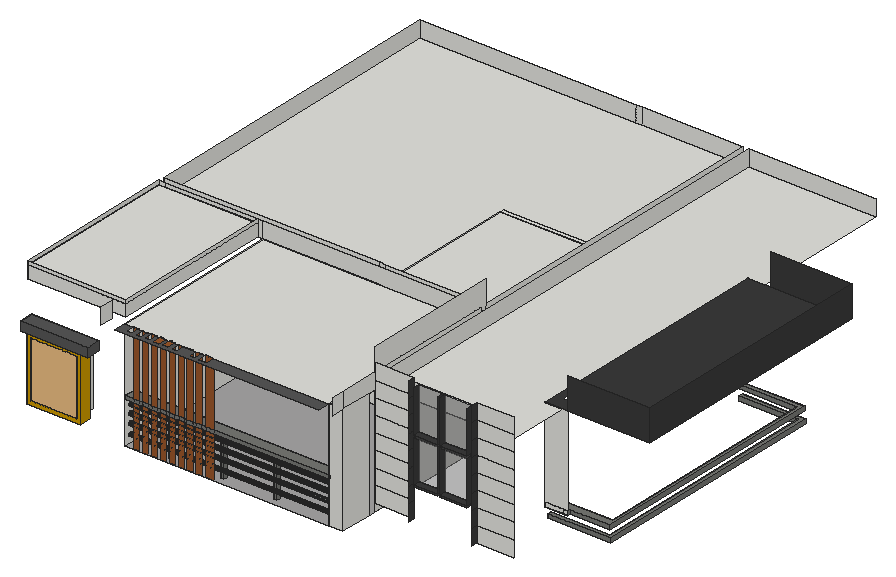
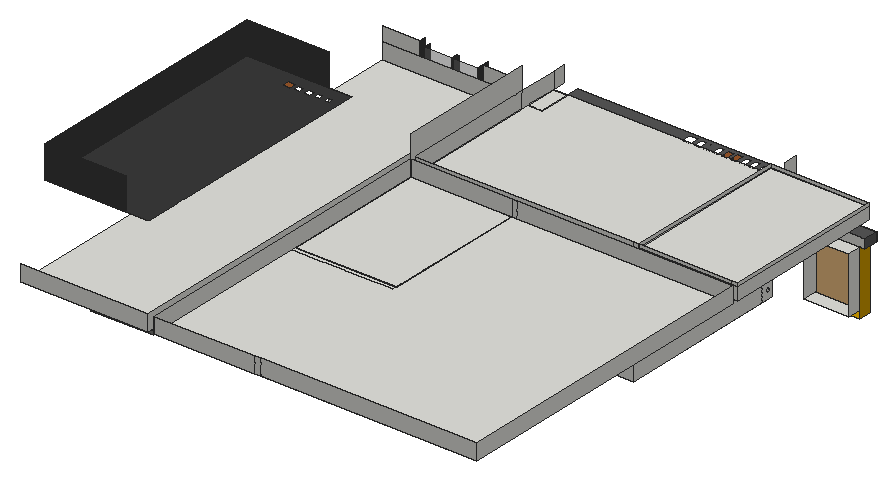
# SketchUp Ruby script. Lengths in inches.
U = 1.inch
M = Sketchup.active_model
def pt(a) = Geom::Point3d.new(a.map { |v| v * U })
def face(e, loops, mat)
  f = e.add_face(loops[0].map { |a| pt(a) })
  loops[1..].each { |l| e.add_face(l.map { |a| pt(a) }).erase! }
  f.material = f.back_material = mat if mat
  f
end
# faces: each face lists its corners as indices into pts; further lists are holes
def faces(e, pts, list, mat = nil) = list.each { |f| face(e, (f[0].is_a?(Array) ? f : [f]).map { |l| l.map { |i| pts[i] } }, mat) }
# xy, xz, yz: faces in a plane at the given z, y or x. An outline is a flat list of corners, or four numbers for a rectangle; further outlines are holes
def ring(l) = l.size == 4 ? [[l[0], l[1]], [l[2], l[1]], [l[2], l[3]], [l[0], l[3]]] : l.each_slice(2).to_a
def flat(e, list, mat, &to3) = list.each { |f| face(e, (f[0].is_a?(Array) ? f : [f]).map { |l| ring(l).map { |u, v| to3.(u, v) } }, mat) }
def xy(e, z, list, mat = nil) = flat(e, list, mat) { |x, y| [x, y, z] }
def xz(e, y, list, mat = nil) = flat(e, list, mat) { |x, z| [x, y, z] }
def yz(e, x, list, mat = nil) = flat(e, list, mat) { |y, z| [x, y, z] }
def lines(e, pts, list) = list.each { |a, b| e.add_line(pt(pts[a]), pt(pts[b])) }
# prism: a flat outline (further loops are holes) pulled along v
def prism(e, loops, v, mat = nil)
  f = face(e, loops, mat); d = Geom::Vector3d.new(v.map { |x| x * U })
  f.pushpull(f.normal.samedirection?(d) ? d.length : -d.length)
end
def box(e, o, s, mat = nil) = prism(e, [[o, [o[0] + s[0], o[1], o[2]], [o[0] + s[0], o[1] + s[1], o[2]], [o[0], o[1] + s[1], o[2]]]], [0, 0, s[2]], mat)
def at(x, y, z, deg = 0) = Geom::Transformation.translation(pt([x, y, z])) * Geom::Transformation.rotation(ORIGIN, Z_AXIS, deg.degrees)
def axes(o, x, y, z) = Geom::Transformation.new([*x, 0, *y, 0, *z, 0, *pt(o).to_a, 1])
def part(name) = M.definitions.add(name)
# library, detail: a bought-in or finely detailed component or shape, given as its bounding box
def library(name, o, s) = part(name).tap { |d| box(d.entities, o, s) }
def detail(e, o, s) = box(e.add_group.entities, o, s)
def put(e, d, t, mat = nil) = e.add_instance(d, t).tap { |i| i.material = mat if mat }
def group(e, t, mat = nil) = e.add_group.tap { |g| g.transformation = t; g.material = mat if mat }.entities
root = M.entities
M.materials.add("[Color C05]").color = [255, 93, 0]
M.materials.add("[Color C08]").color = [74, 47, 0]
M.materials.add("[Color D06]").color = [204, 153, 0]
M.materials.add("[Color M06]").color = [86, 86, 86]
M.materials.add("[Color M07]").color = [58, 58, 58]
M.materials.add("[Metal Seamed]").color = [118, 119, 115]
M.materials.add("[Stone Vein Gray]").color = [166, 165, 165]
M.materials.add("[Translucent Glass Gray]").color = [128, 128, 128]
M.materials["[Translucent Glass Gray]"].alpha = 0.5
M.materials.add("[Wood Cherry Original]").color = [152, 86, 42]
c1 = part("Group\#3")
xy(c1.entities,0,[[0,0,48,8.5625]],"[Color C08]")
xy(c1.entities,4.98,[[4.98,0,43.02,2.5625],[4.98,2.5625,43.02,8.5625]],"[Color C08]")
xy(c1.entities,79.02,[[4.98,0,43.02,2.5625],[4.98,2.5625,43.02,8.5625]],"[Color C08]")
xy(c1.entities,84,[[0,0,48,8.5625]],"[Color C08]")
xz(c1.entities,0,[[[0,0,48,84],[4.98,4.98,43.02,79.02]]],"[Color C08]")
xz(c1.entities,2.5625,[[4.98,4.98,43.02,79.02]],"[Color C05]")
xz(c1.entities,8.5625,[[[0,0,48,84],[4.98,4.98,43.02,79.02]]],"[Color C08]")
yz(c1.entities,0,[[0,0,8.5625,84]],"[Color C08]")
yz(c1.entities,4.98,[[0,4.98,2.5625,79.02],[2.5625,4.98,8.5625,79.02]],"[Color C08]")
yz(c1.entities,43.02,[[0,4.98,2.5625,79.02],[2.5625,4.98,8.5625,79.02]],"[Color C08]")
yz(c1.entities,48,[[0,0,8.5625,84]],"[Color C08]")
c2 = library("Group\#4",[0,0,0],[48,6,60])
xy(root,164.875,[[336.97,106.4375,352,140.0625]])
xy(root,164.875,[[273.15,113.09,276.47,116.4]],"[Metal Seamed]")
xy(root,164.875,[[[120,106.4375,336.97,106.4375,336.97,140.0625,352,140.0625,352,449.1875,322.29,449.1875,322.29,453.4375,274.29,453.4375,274.29,449.1875,244.75,449.1875,244.75,290.0625,120,290.0625],[161.28,113.09,164.59,116.4],[216.4,113.09,219.72,116.4],[273.15,113.09,276.47,116.4]]],"[Stone Vein Gray]")
xy(root,169.04,[[475.4375,224.05,475.4375,228.48,537.83,228.48,537.83,478.41,475.4375,478.41,475.4375,483.17,542.5625,483.17,542.5625,224.05]],"[Metal Seamed]")
xy(root,173.48,[[475.4375,224.05,542.5625,224.05,542.5625,483.17,475.4375,483.17,475.4375,478.41,537.83,478.41,537.83,228.48,475.4375,228.48]],"[Metal Seamed]")
xy(root,176.87,[[25.93,93.75,82.74,106.4375]],"[Color D06]")
xy(root,179.95,[[180.25,290.0625,233.4375,296.0625]])
xy(root,181.27,[[30.34,93.75,78.34,115.4375]])
xy(root,181.87,[[475.4375,220.28,475.4375,231.31,538.41,231.31,538.41,476.42,541.89,476.42,541.89,481.18,542.5625,481.18,542.5625,222.97,500,222.97,500,220.28],[475.4375,476.33,475.4375,481.18,534.52,481.18,534.52,480.67,536.58,480.67,536.58,476.33],[536.58,476.33,538.41,476.42],[536.58,476.42,541.89,480.67],[534.52,480.67,541.89,481.18]],"[Metal Seamed]")
xy(root,182.4375,[[536.02,226.32,541.65,232.26]],"[Metal Seamed]")
xy(root,186.3125,[[475.4375,220.28,500,220.28,500,222.97,542.5625,222.97,542.5625,481.18,475.4375,481.18,475.4375,476.33,538.41,476.33,538.41,231.31,475.4375,231.31]],"[Metal Seamed]")
xy(root,208.4375,[[216.4,113.09,219.72,116.4]],"[Metal Seamed]")
xy(root,208.53,[[399.25,141.23,424.3125,147.79],[427.08,141.23,456,147.79]],"[Color M07]")
xy(root,209.16,[[336.97,106.4375,337.375,118.875],[336.97,118.875,337.375,140.0625]])
xy(root,209.16,[[[120,106.4375,336.97,118.875],[161.28,113.09,164.59,116.4],[273.15,113.09,276.47,116.4]]],"[Metal Seamed]")
xy(root,210.6,[[399.25,141.23,424.3125,147.79],[427.08,141.23,456,147.79]],"[Color M07]")
xy(root,212.875,[[336.97,106.4375,337.375,118.875],[336.97,118.875,337.375,140.0625]])
xy(root,212.875,[[120,106.4375,336.97,118.875]],"[Metal Seamed]")
xy(root,241.27,[[30.34,93.75,78.34,115.4375]])
xy(root,245.68,[[25.93,93.75,82.74,106.4375]])
xy(root,245.68,[[20.68,91.3125,20.68,106.4375,25.93,106.4375,25.93,93.75,82.74,93.75,82.74,106.4375,92.11,106.4375,92.11,91.3125]],"[Color M06]")
xy(root,248.875,[[274.29,449.1875,322.29,453.4375]])
xy(root,251.14,[[180.25,290.0625,233.4375,296.0625]])
xy(root,255.3,[[20.68,91.3125,92.11,106.4375]],"[Color M06]")
xy(root,255.4,[[399.25,141.23,424.3125,147.79],[427.08,141.23,456,147.79]],"[Color M07]")
xy(root,257.48,[[399.25,141.23,424.3125,147.79],[427.08,141.23,456,147.79]],"[Color M07]")
xy(root,280.8125,[[186.11,97.4375,191.67,106.4375]],"[Wood Cherry Original]")
xy(root,281,[[120,106.4375,120,290.0625,352,290.0625,352,140.0625,336.97,140.0625,336.97,106.4375],[336.97,106.4375,352,140.0625],[358,155.92,494,155.92,494,220.28,475.4375,220.28,475.4375,489.49,494,489.49,494,637.4375,358,637.4375],[244.75,290.0625,352,296.0625],[9,296.0625,244.75,296.0625,244.75,453.4375,352,453.4375,352,637.4375,9,637.4375],
  [244.75,296.0625,352,449.1875],[244.75,449.1875,352,453.4375]])
xy(root,281,[[120,92.4375,120,106.4375,129.11,106.4375,129.11,97.4375,134.67,97.4375,134.67,106.4375,138.61,106.4375,138.61,97.4375,144.17,97.4375,144.17,106.4375,148.11,106.4375,148.11,97.4375,153.67,97.4375,153.67,106.4375,176.61,106.4375,176.61,97.4375,182.17,97.4375,182.17,106.4375,195.61,106.4375,195.61,97.4375,201.17,97.4375,201.17,106.4375,205.34,106.4375,205.34,96.98,214.79,96.98,214.79,106.4375,336.97,106.4375,336.97,92.4375]],"[Color M06]")
xy(root,281,[[[475.4375,220.28,586.5,489.49],[514.62,234.2,520.93,240.63],[482.87,234.2,489.18,240.63],[503.93,234.2,510.24,240.63],[493.55,234.2,499.87,240.57]]],"[Color M07]")
xy(root,281.125,[[167.11,97.4375,172.67,106.4375]],"[Wood Cherry Original]")
xy(root,281.1875,[[525.05,234.2,531.37,240.63]],"[Wood Cherry Original]")
xy(root,281.25,[[157.61,97.4375,163.17,106.4375]],"[Wood Cherry Original]")
xy(root,294,[[9,115.4375,114,290.0625]])
xz(root,91.3125,[[20.68,245.68,92.11,255.3]],"[Color M06]")
xz(root,93.75,[[[25.93,176.87,82.74,245.68],[30.34,181.27,78.34,241.27]]],"[Color D06]")
xz(root,106.4375,[[336.97,164.875,352,164.875,352,281,336.97,281,336.97,212.875,337.375,212.875,337.375,209.16,336.97,209.16],[336.97,209.16,337.375,212.875],[20.68,245.68,92.11,255.3],[157.61,281,163.17,281.25],[167.11,281,172.67,281.125]])
xz(root,106.4375,[[120,209.16,129.11,212.875],[129.11,209.16,134.67,212.875],[134.67,209.16,138.61,212.875],[138.61,209.16,144.17,212.875],[144.17,209.16,148.11,212.875],
  [148.11,209.16,153.67,212.875],[153.67,209.16,157.61,212.875],[157.61,209.16,163.17,212.875],[163.17,209.16,167.11,212.875],[167.11,209.16,172.67,212.875],
  [172.67,209.16,176.61,212.875],[176.61,209.16,182.17,212.875],[182.17,209.16,186.11,212.875],[186.11,209.16,191.67,212.875],[191.67,209.16,195.61,212.875],
  [195.61,209.16,201.17,212.875],[201.17,209.16,205.34,212.875],[205.34,209.16,214.79,212.875],[214.79,209.16,336.97,212.875]],"[Metal Seamed]")
xz(root,106.4375,[[129.11,164.875,134.67,209.16],[138.61,164.875,144.17,209.16],[148.11,164.875,153.67,209.16],[157.61,164.875,163.17,209.16],[167.11,164.875,172.67,209.16],
  [176.61,164.875,182.17,209.16],[186.11,164.875,191.67,209.16],[195.61,164.875,201.17,209.16],[205.34,164.875,214.79,209.16],[129.11,212.875,134.67,281],
  [138.61,212.875,144.17,281],[148.11,212.875,153.67,281],[157.61,212.875,163.17,281],[167.11,212.875,172.67,281],[176.61,212.875,182.17,281],
  [186.11,212.875,191.67,280.8125],[195.61,212.875,201.17,281],[205.34,212.875,214.79,281]],"[Wood Cherry Original]")
xz(root,113.09,[[161.28,164.875,164.59,209.16],[216.4,164.875,219.72,208.4375],[273.15,164.875,276.47,209.16]],"[Metal Seamed]")
xz(root,115.4375,[[9,281,114,294],[9,294,114,298]])
xz(root,116.4,[[161.28,164.875,164.59,209.16],[216.4,164.875,219.72,208.4375],[273.15,164.875,276.47,209.16]],"[Metal Seamed]")
xz(root,118.875,[[120,209.16,337.375,212.875]],"[Metal Seamed]")
xz(root,140.0625,[[336.97,164.875,336.97,209.16,337.375,209.16,337.375,212.875,336.97,212.875,336.97,281,352,281,352,164.875]])
xz(root,147.79,[[352,173.6,394.33,190.35],[460.92,173.6,500,190.35],[352,190.35,394.33,207.1],[460.92,190.35,500,207.1],[352,207.1,394.33,223.85],
  [460.92,207.1,500,223.85],[352,223.85,394.33,240.6],[460.92,223.85,500,240.6],[352,240.6,394.33,257.35],[460.92,240.6,500,257.35],
  [352,257.35,394.33,274.1],[460.92,257.35,500,274.1],[352,274.1,394.33,290.85],[460.92,274.1,500,290.85],[352,290.85,394.33,307.6],
  [460.92,290.85,500,307.6]])
xz(root,147.79,[[399.25,210.6,424.3125,255.4],[427.08,210.6,456,255.4],[399.25,257.48,424.3125,302.9],[427.08,257.48,456,302.9]],"[Translucent Glass Gray]")
xz(root,155.92,[[358,281,494,298]])
xz(root,220.28,[[475.4375,181.87,494,186.3125],[494,181.87,500,186.3125],[475.4375,186.3125,500,281]])
xz(root,220.28,[[500,281,586.5,315]],"[Color M07]")
xz(root,222.97,[[500,181.87,542.5625,186.3125]],"[Metal Seamed]")
xz(root,224.05,[[475.4375,169.04,542.5625,173.48]],"[Metal Seamed]")
xz(root,228.48,[[475.4375,169.04,537.83,173.48]],"[Metal Seamed]")
xz(root,231.31,[[475.4375,181.87,538.41,186.3125]],"[Metal Seamed]")
xz(root,290.0625,[[[120,164.875,244.75,281],[180.25,179.95,233.4375,251.14]],[9,281,114,294],[114,281,120,298],[120,281,352,298],[9,294,15,298],
  [15,294,114,298]])
xz(root,296.0625,[[9,281,238.75,298],[238.75,281,244.75,298],[244.75,281,352,298]])
xz(root,449.1875,[[244.75,164.875,274.29,164.875,274.29,248.875,322.29,248.875,322.29,164.875,352,164.875,352,281,244.75,281]])
xz(root,476.33,[[475.4375,181.87,538.41,186.3125]],"[Metal Seamed]")
xz(root,478.41,[[475.4375,169.04,537.83,173.48]],"[Metal Seamed]")
xz(root,481.18,[[475.4375,181.87,542.5625,186.3125]],"[Metal Seamed]")
xz(root,483.17,[[475.4375,169.04,542.5625,173.48]],"[Metal Seamed]")
xz(root,489.49,[[500,281,586.5,315]],"[Color M07]")
xz(root,637.4375,[[9,281,238.75,298],[238.75,281,244.75,298],[244.75,281,352,298],[358,281,494,298]])
yz(root,9,[[115.4375,281,290.0625,294],[296.0625,281,637.4375,298],[115.4375,294,290.0625,298]])
yz(root,20.68,[[91.3125,245.68,106.4375,255.3]],"[Color M06]")
yz(root,25.93,[[93.75,176.87,106.4375,245.68]],"[Color D06]")
yz(root,30.34,[[93.75,181.27,115.4375,241.27]])
yz(root,78.34,[[93.75,181.27,115.4375,241.27]])
yz(root,82.74,[[93.75,176.87,106.4375,245.68]],"[Color D06]")
yz(root,92.11,[[91.3125,245.68,106.4375,255.3]],"[Color M06]")
yz(root,105.8,[[92.4375,281,106.4375,298]])
yz(root,114,[[115.4375,281,290.0625,294],[115.4375,294,290.0625,298]])
yz(root,120,[[118.875,164.875,290.0625,164.875,290.0625,281,106.4375,281,106.4375,212.875,118.875,212.875],[[106.4375,164.875,118.875,209.16],[112.14,191.67,111.69,191.73,111.27,191.9,110.91,192.18,110.63,192.54,110.45,192.96,110.39,193.42,110.45,193.87,110.63,194.29,110.91,194.65,111.27,194.93,111.69,195.11,112.14,195.17,112.6,195.11,113.02,194.93,113.38,194.65,113.66,194.29,113.83,193.87,113.89,193.42,113.83,192.96,113.66,192.54,113.38,192.18,113.02,191.9,112.6,191.73],[112.14,182.23,111.69,182.29,111.27,182.46,110.91,182.74,110.63,183.1,110.45,183.53,110.39,183.98,110.45,184.43,110.63,184.85,110.91,185.22,111.27,185.49,111.69,185.67,112.14,185.73,112.6,185.67,113.02,185.49,113.38,185.22,113.66,184.85,113.83,184.43,113.89,183.98,113.83,183.53,113.66,183.1,113.38,182.74,113.02,182.46,112.6,182.29],[112.14,172.04,111.69,172.1,111.27,172.28,110.91,172.55,110.63,172.92,110.45,173.34,110.39,173.79,110.45,174.24,110.63,174.67,110.91,175.03,111.27,175.31,111.69,175.48,112.14,175.54,112.6,175.48,113.02,175.31,113.38,175.03,113.66,174.67,113.83,174.24,113.89,173.79,113.83,173.34,113.66,172.92,113.38,172.55,113.02,172.28,112.6,172.1],[112.14,200.85,111.69,200.91,111.27,201.09,110.91,201.37,110.63,201.73,110.45,202.15,110.39,202.6,110.45,203.06,110.63,203.48,110.91,203.84,111.27,204.12,111.69,204.29,112.14,204.35,112.6,204.29,113.02,204.12,113.38,203.84,113.66,203.48,113.83,203.06,113.89,202.6,113.83,202.15,113.66,201.73,113.38,201.37,113.02,201.09,112.6,200.91]],[112.14,172.04,111.69,172.1,111.27,172.28,110.91,172.55,110.63,172.92,110.45,173.34,110.39,173.79,110.45,174.24,110.63,174.67,110.91,175.03,111.27,175.31,111.69,175.48,112.14,175.54,112.6,175.48,113.02,175.31,113.38,175.03,113.66,174.67,113.83,174.24,113.89,173.79,113.83,173.34,113.66,172.92,113.38,172.55,113.02,172.28,112.6,172.1],[112.14,182.23,111.69,182.29,111.27,182.46,110.91,182.74,110.63,183.1,110.45,183.53,110.39,183.98,110.45,184.43,110.63,184.85,110.91,185.22,111.27,185.49,111.69,185.67,112.14,185.73,112.6,185.67,113.02,185.49,113.38,185.22,113.66,184.85,113.83,184.43,113.89,183.98,113.83,183.53,113.66,183.1,113.38,182.74,113.02,182.46,112.6,182.29],[112.14,191.67,111.69,191.73,111.27,191.9,110.91,192.18,110.63,192.54,110.45,192.96,110.39,193.42,110.45,193.87,110.63,194.29,110.91,194.65,111.27,194.93,111.69,195.11,112.14,195.17,112.6,195.11,113.02,194.93,113.38,194.65,113.66,194.29,113.83,193.87,113.89,193.42,113.83,192.96,113.66,192.54,113.38,192.18,113.02,191.9,112.6,191.73],
  [112.14,200.85,111.69,200.91,111.27,201.09,110.91,201.37,110.63,201.73,110.45,202.15,110.39,202.6,110.45,203.06,110.63,203.48,110.91,203.84,111.27,204.12,111.69,204.29,112.14,204.35,112.6,204.29,113.02,204.12,113.38,203.84,113.66,203.48,113.83,203.06,113.89,202.6,113.83,202.15,113.66,201.73,113.38,201.37,113.02,201.09,112.6,200.91],[106.4375,209.16,118.875,212.875]])
yz(root,161.28,[[113.09,164.875,116.4,209.16]],"[Metal Seamed]")
yz(root,164.59,[[113.09,164.875,116.4,209.16]],"[Metal Seamed]")
yz(root,180.25,[[290.0625,179.95,296.0625,251.14]])
yz(root,216.4,[[113.09,164.875,116.4,208.4375]],"[Metal Seamed]")
yz(root,219.72,[[113.09,164.875,116.4,208.4375]],"[Metal Seamed]")
yz(root,233.4375,[[290.0625,179.95,296.0625,251.14]])
yz(root,244.75,[[290.0625,164.875,296.0625,281],[296.0625,164.875,449.1875,281]])
yz(root,273.15,[[113.09,164.875,116.4,209.16]],"[Metal Seamed]")
yz(root,274.29,[[449.1875,164.875,453.4375,248.875]])
yz(root,276.47,[[113.09,164.875,116.4,209.16]],"[Metal Seamed]")
yz(root,322.29,[[449.1875,164.875,453.4375,248.875]])
yz(root,336.9375,[[112.14,191.67,112.6,191.73,113.02,191.9,113.38,192.18,113.66,192.54,113.83,192.96,113.89,193.42,113.83,193.87,113.66,194.29,113.38,194.65,113.02,194.93,112.6,195.11,112.14,195.17,111.69,195.11,111.27,194.93,110.91,194.65,110.63,194.29,110.45,193.87,110.39,193.42,110.45,192.96,110.63,192.54,110.91,192.18,111.27,191.9,111.69,191.73]])
yz(root,336.97,[[[106.4375,164.875,140.0625,209.16],[112.14,200.85,112.6,200.91,113.02,201.09,113.38,201.37,113.66,201.73,113.83,202.15,113.89,202.6,113.83,203.06,113.66,203.48,113.38,203.84,113.02,204.12,112.6,204.29,112.14,204.35,111.69,204.29,111.27,204.12,110.91,203.84,110.63,203.48,110.45,203.06,110.39,202.6,110.45,202.15,110.63,201.73,110.91,201.37,111.27,201.09,111.69,200.91]],[106.4375,212.875,140.0625,281]])
yz(root,337.375,[[106.4375,209.16,118.875,212.875],[118.875,209.16,140.0625,212.875]])
yz(root,337.5625,[[112.14,182.23,112.6,182.29,113.02,182.46,113.38,182.74,113.66,183.1,113.83,183.53,113.89,183.98,113.83,184.43,113.66,184.85,113.38,185.22,113.02,185.49,112.6,185.67,112.14,185.73,111.69,185.67,111.27,185.49,110.91,185.22,110.63,184.85,110.45,184.43,110.39,183.98,110.45,183.53,110.63,183.1,110.91,182.74,111.27,182.46,111.69,182.29]])
yz(root,340.4375,[[112.14,172.04,112.6,172.1,113.02,172.28,113.38,172.55,113.66,172.92,113.83,173.34,113.89,173.79,113.83,174.24,113.66,174.67,113.38,175.03,113.02,175.31,112.6,175.48,112.14,175.54,111.69,175.48,111.27,175.31,110.91,175.03,110.63,174.67,110.45,174.24,110.39,173.79,110.45,173.34,110.63,172.92,110.91,172.55,111.27,172.28,111.69,172.1]])
yz(root,352,[[106.4375,164.875,140.0625,281],[147.79,164.875,449.1875,281],[92.4375,281,106.4375,298],[106.4375,281,147.79,298],[147.79,281,290.0625,298],
  [290.0625,281,290.0625,298,147.79,298,147.79,322,296.0625,322,296.0625,281],[296.0625,281,637.4375,298]])
yz(root,358,[[155.92,281,637.4375,298]])
yz(root,394.33,[[141.23,173.6,147.79,190.35],[141.23,190.35,147.79,207.1],[141.23,207.1,147.79,223.85],[141.23,223.85,147.79,240.6],[141.23,240.6,147.79,257.35],
  [141.23,257.35,147.79,274.1],[141.23,274.1,147.79,290.85],[141.23,290.85,147.79,307.6]],"[Color M07]")
yz(root,399.25,[[141.23,210.6,147.79,255.4],[141.23,257.48,147.79,302.9]],"[Color M07]")
yz(root,424.3125,[[141.23,210.6,147.79,255.4],[141.23,257.48,147.79,302.9]],"[Color M07]")
yz(root,427.08,[[141.23,210.6,147.79,255.4],[141.23,257.48,147.79,302.9]],"[Color M07]")
yz(root,456,[[141.23,210.6,147.79,255.4],[141.23,257.48,147.79,302.9]],"[Color M07]")
yz(root,460.92,[[141.23,173.6,147.79,190.35],[141.23,190.35,147.79,207.1],[141.23,207.1,147.79,223.85],[141.23,223.85,147.79,240.6],[141.23,240.6,147.79,257.35],
  [141.23,257.35,147.79,274.1],[141.23,274.1,147.79,290.85],[141.23,290.85,147.79,307.6]],"[Color M07]")
yz(root,475.4375,[[224.05,169.04,228.48,173.48],[220.28,181.87,231.31,186.3125]])
yz(root,500,[[220.28,181.87,222.97,186.3125]],"[Metal Seamed]")
yz(root,537.83,[[228.48,169.04,478.41,173.48]],"[Metal Seamed]")
yz(root,538.41,[[231.31,181.87,476.33,186.3125]],"[Metal Seamed]")
yz(root,542.5625,[[224.05,169.04,483.17,173.48],[222.97,181.87,481.18,186.3125]],"[Metal Seamed]")
yz(root,586.5,[[220.28,281,489.49,315]],"[Color M07]")
p = [[120,111.69,172.1],[120,112.14,172.04],[340.4375,112.14,172.04],[340.4375,111.69,172.1],[120,112.6,172.1],[340.4375,112.6,172.1],
  [120,111.27,172.28],[340.4375,111.27,172.28],[120,113.02,172.28],[340.4375,113.02,172.28],[120,110.91,172.55],[340.4375,110.91,172.55],
  [120,113.38,172.55],[340.4375,113.38,172.55],[120,110.63,172.92],[340.4375,110.63,172.92],[120,113.66,172.92],[340.4375,113.66,172.92],
  [120,110.45,173.34],[340.4375,110.45,173.34],[120,113.83,173.34],[340.4375,113.83,173.34],[120,110.39,173.79],[340.4375,110.39,173.79],
  [120,113.89,173.79],[340.4375,113.89,173.79],[120,110.45,174.24],[340.4375,110.45,174.24],[120,113.83,174.24],[340.4375,113.83,174.24],
  [120,110.63,174.67],[340.4375,110.63,174.67],[120,113.66,174.67],[340.4375,113.66,174.67],[120,110.91,175.03],[340.4375,110.91,175.03],
  [120,113.38,175.03],[340.4375,113.38,175.03],[120,111.27,175.31],[340.4375,111.27,175.31],[120,113.02,175.31],[340.4375,113.02,175.31],
  [120,111.69,175.48],[340.4375,111.69,175.48],[120,112.6,175.48],[340.4375,112.6,175.48],[120,112.14,175.54],[340.4375,112.14,175.54],
  [120,111.69,182.29],[120,112.14,182.23],[337.5625,112.14,182.23],[337.5625,111.69,182.29],[120,112.6,182.29],[337.5625,112.6,182.29],
  [120,111.27,182.46],[337.5625,111.27,182.46],[120,113.02,182.46],[337.5625,113.02,182.46],[120,110.91,182.74],[337.5625,110.91,182.74],
  [120,113.38,182.74],[337.5625,113.38,182.74],[120,110.63,183.1],[337.5625,110.63,183.1],[120,113.66,183.1],[337.5625,113.66,183.1],
  [120,110.45,183.53],[337.5625,110.45,183.53],[120,113.83,183.53],[337.5625,113.83,183.53],[120,110.39,183.98],[337.5625,110.39,183.98],
  [120,113.89,183.98],[337.5625,113.89,183.98],[120,110.45,184.43],[337.5625,110.45,184.43],[120,113.83,184.43],[337.5625,113.83,184.43],
  [120,110.63,184.85],[337.5625,110.63,184.85],[120,113.66,184.85],[337.5625,113.66,184.85],[120,110.91,185.22],[337.5625,110.91,185.22],
  [120,113.38,185.22],[337.5625,113.38,185.22],[120,111.27,185.49],[337.5625,111.27,185.49],[120,113.02,185.49],[337.5625,113.02,185.49],
  [120,111.69,185.67],[337.5625,111.69,185.67],[120,112.6,185.67],[337.5625,112.6,185.67],[120,112.14,185.73],[337.5625,112.14,185.73],
  [120,111.27,191.9],[120,111.69,191.73],[336.9375,111.69,191.73],[336.9375,111.27,191.9],[120,112.14,191.67],[336.9375,112.14,191.67],
  [120,112.6,191.73],[336.9375,112.6,191.73],[120,113.02,191.9],[336.9375,113.02,191.9],[120,110.91,192.18],[336.9375,110.91,192.18],
  [120,113.38,192.18],[336.9375,113.38,192.18],[120,110.63,192.54],[336.9375,110.63,192.54],[120,113.66,192.54],[336.9375,113.66,192.54],
  [120,110.45,192.96],[336.9375,110.45,192.96],[120,113.83,192.96],[336.9375,113.83,192.96],[120,110.39,193.42],[336.9375,110.39,193.42],
  [120,113.89,193.42],[336.9375,113.89,193.42],[120,110.45,193.87],[336.9375,110.45,193.87],[120,113.83,193.87],[336.9375,113.83,193.87],
  [120,110.63,194.29],[336.9375,110.63,194.29],[120,113.66,194.29],[336.9375,113.66,194.29],[120,110.91,194.65],[336.9375,110.91,194.65],
  [120,113.38,194.65],[336.9375,113.38,194.65],[120,111.27,194.93],[336.9375,111.27,194.93],[120,113.02,194.93],[336.9375,113.02,194.93],
  [120,111.69,195.11],[336.9375,111.69,195.11],[120,112.6,195.11],[336.9375,112.6,195.11],[120,112.14,195.17],[336.9375,112.14,195.17],
  [120,111.27,201.09],[120,111.69,200.91],[336.97,111.69,200.91],[336.97,111.27,201.09],[120,112.14,200.85],[336.97,112.14,200.85],
  [120,112.6,200.91],[336.97,112.6,200.91],[120,113.02,201.09],[336.97,113.02,201.09],[120,110.91,201.37],[336.97,110.91,201.37],
  [120,113.38,201.37],[336.97,113.38,201.37],[120,110.63,201.73],[336.97,110.63,201.73],[120,113.66,201.73],[336.97,113.66,201.73],
  [120,110.45,202.15],[336.97,110.45,202.15],[120,113.83,202.15],[336.97,113.83,202.15],[120,110.39,202.6],[336.97,110.39,202.6],
  [120,113.89,202.6],[336.97,113.89,202.6],[120,110.45,203.06],[336.97,110.45,203.06],[120,113.83,203.06],[336.97,113.83,203.06],
  [120,110.63,203.48],[336.97,110.63,203.48],[120,113.66,203.48],[336.97,113.66,203.48],[120,110.91,203.84],[336.97,110.91,203.84],
  [120,113.38,203.84],[336.97,113.38,203.84],[120,111.27,204.12],[336.97,111.27,204.12],[120,113.02,204.12],[336.97,113.02,204.12],
  [120,111.69,204.29],[336.97,111.69,204.29],[120,112.6,204.29],[336.97,112.6,204.29],[120,112.14,204.35],[336.97,112.14,204.35]]
faces(root,p,[[0,1,2,3],[1,4,5,2],[6,0,3,7],[4,8,9,5],[10,6,7,11],[8,12,13,9],[14,10,11,15],[12,16,17,13],
  [18,14,15,19],[16,20,21,17],[22,18,19,23],[20,24,25,21],[26,22,23,27],[24,28,29,25],[30,26,27,31],[28,32,33,29],
  [34,30,31,35],[32,36,37,33],[38,34,35,39],[36,40,41,37],[42,38,39,43],[40,44,45,41],[46,42,43,47],[44,46,47,45],
  [48,49,50,51],[49,52,53,50],[54,48,51,55],[52,56,57,53],[58,54,55,59],[56,60,61,57],[62,58,59,63],[60,64,65,61],
  [66,62,63,67],[64,68,69,65],[70,66,67,71],[68,72,73,69],[74,70,71,75],[72,76,77,73],[78,74,75,79],[76,80,81,77],
  [82,78,79,83],[80,84,85,81],[86,82,83,87],[84,88,89,85],[90,86,87,91],[88,92,93,89],[94,90,91,95],[92,94,95,93],
  [96,97,98,99],[97,100,101,98],[100,102,103,101],[102,104,105,103],[106,96,99,107],[104,108,109,105],[110,106,107,111],[108,112,113,109],
  [114,110,111,115],[112,116,117,113],[118,114,115,119],[116,120,121,117],[122,118,119,123],[120,124,125,121],[126,122,123,127],[124,128,129,125],
  [130,126,127,131],[128,132,133,129],[134,130,131,135],[132,136,137,133],[138,134,135,139],[136,140,141,137],[142,138,139,143],[140,142,143,141],
  [144,145,146,147],[145,148,149,146],[148,150,151,149],[150,152,153,151],[154,144,147,155],[152,156,157,153],[158,154,155,159],[156,160,161,157],
  [162,158,159,163],[160,164,165,161],[166,162,163,167],[164,168,169,165],[170,166,167,171],[168,172,173,169],[174,170,171,175],[172,176,177,173],
  [178,174,175,179],[176,180,181,177],[182,178,179,183],[180,184,185,181],[186,182,183,187],[184,188,189,185],[190,186,187,191],[188,190,191,189]],"[Metal Seamed]")
put(root,c1,at(274.29,449.1875,164.875))
put(root,c2,axes([180.25,290.0625,179.95],[1.10807,0,0],[0,0.87,0],[0,0,1.18646]))
put(root,c2,at(30.34,93.75,181.27))
